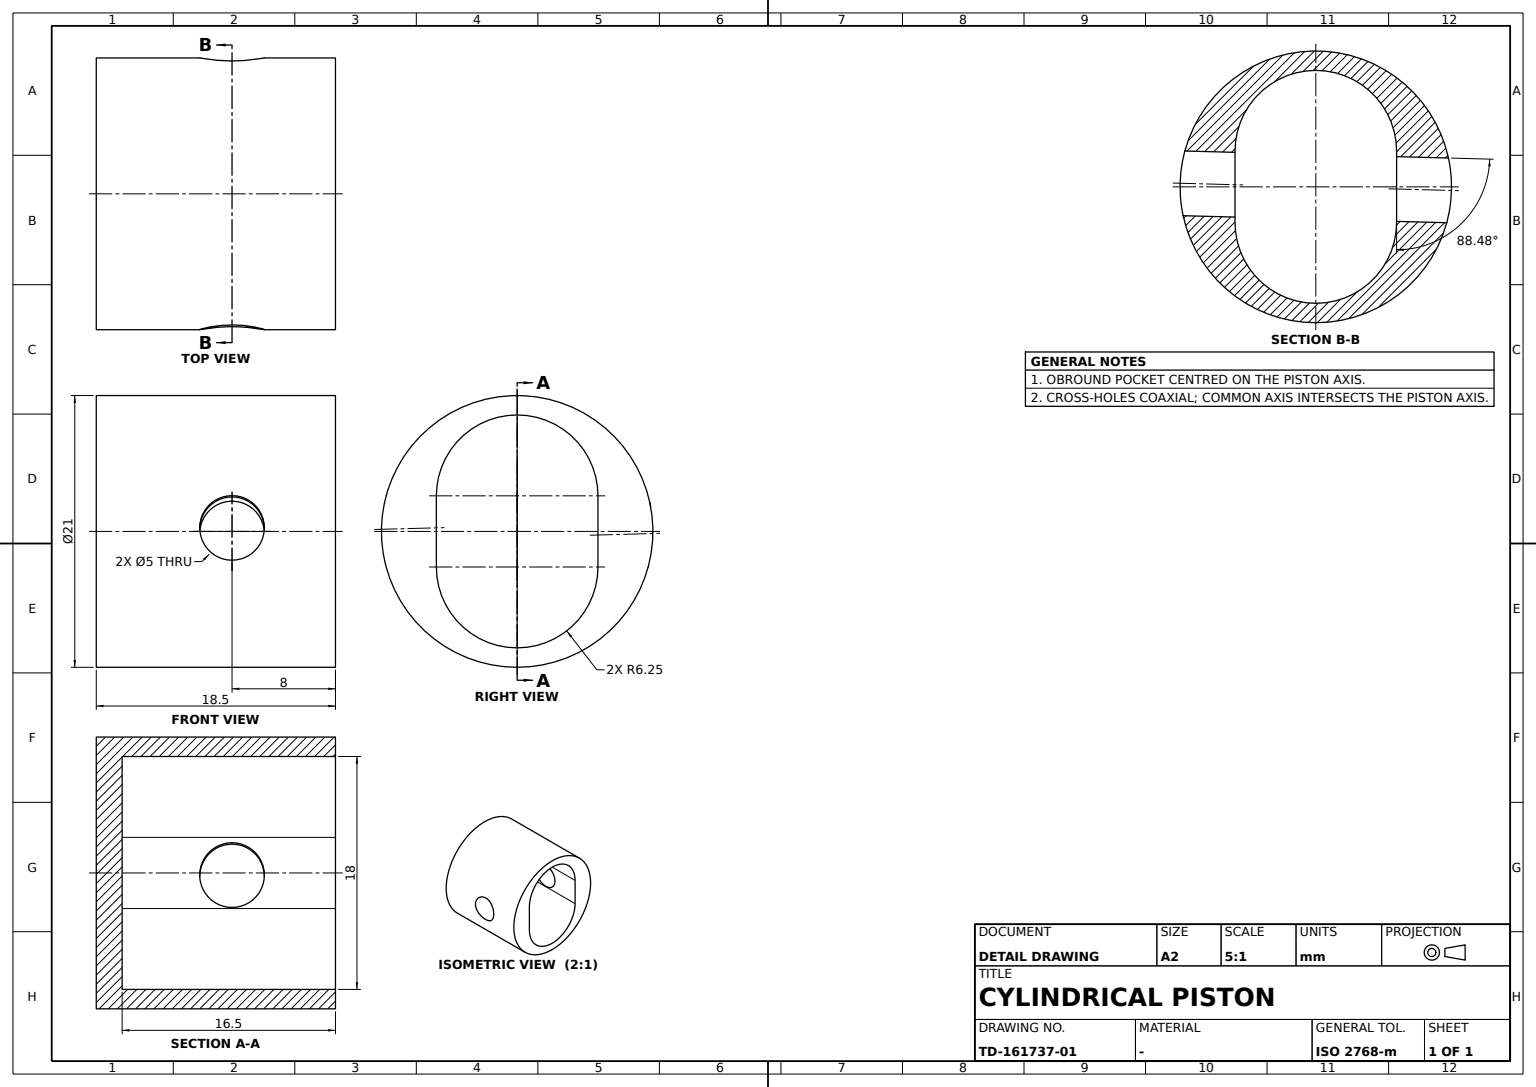
ISO-10303-21;
HEADER;
FILE_DESCRIPTION((''),'2;1');
FILE_NAME('','',(''),(''),'','','');
FILE_SCHEMA(('AUTOMOTIVE_DESIGN'));
ENDSEC;
DATA;
#1=APPLICATION_CONTEXT('');
#2=PRODUCT_CONTEXT('',#1,'mechanical');
#3=PRODUCT('','','',(#2));
#4=PRODUCT_DEFINITION_FORMATION('','',#3);
#5=PRODUCT_DEFINITION_CONTEXT('',#1,'design');
#6=PRODUCT_DEFINITION('','',#4,#5);
#7=PRODUCT_DEFINITION_SHAPE('','',#6);
#8=(LENGTH_UNIT()NAMED_UNIT(*)SI_UNIT(.MILLI.,.METRE.));
#9=(NAMED_UNIT(*)PLANE_ANGLE_UNIT()SI_UNIT($,.RADIAN.));
#10=(NAMED_UNIT(*)SI_UNIT($,.STERADIAN.)SOLID_ANGLE_UNIT());
#11=UNCERTAINTY_MEASURE_WITH_UNIT(LENGTH_MEASURE(0.005),#8,'distance_accuracy_value','');
#12=(GEOMETRIC_REPRESENTATION_CONTEXT(3)GLOBAL_UNCERTAINTY_ASSIGNED_CONTEXT((#11))GLOBAL_UNIT_ASSIGNED_CONTEXT((#8,#9,#10))REPRESENTATION_CONTEXT('',''));
#13=CARTESIAN_POINT('',(-2.75,6.25,-16.5));
#14=VERTEX_POINT('',#13);
#15=CARTESIAN_POINT('',(-2.75,-6.25,-16.5));
#16=VERTEX_POINT('',#15);
#17=CARTESIAN_POINT('',(-2.75,0.,-16.5));
#18=DIRECTION('',(0.,0.,1.));
#19=DIRECTION('',(1.,0.,0.));
#20=AXIS2_PLACEMENT_3D('',#17,#18,#19);
#21=CIRCLE('',#20,6.25);
#22=EDGE_CURVE('',#14,#16,#21,.T.);
#23=ORIENTED_EDGE('',*,*,#22,.F.);
#24=CARTESIAN_POINT('',(-2.75,6.25,0.));
#25=VERTEX_POINT('',#24);
#26=CARTESIAN_POINT('',(-2.75,6.25,-8.25));
#27=VECTOR('',#18,1000.);
#28=LINE('',#26,#27);
#29=EDGE_CURVE('',#25,#14,#28,.F.);
#30=ORIENTED_EDGE('',*,*,#29,.F.);
#31=CARTESIAN_POINT('',(-2.75,-6.25,0.));
#32=VERTEX_POINT('',#31);
#33=CARTESIAN_POINT('',(-2.75,0.,0.));
#34=AXIS2_PLACEMENT_3D('',#33,#18,#19);
#35=CIRCLE('',#34,6.25);
#36=EDGE_CURVE('',#25,#32,#35,.T.);
#37=ORIENTED_EDGE('',*,*,#36,.T.);
#38=CARTESIAN_POINT('',(-2.75,-6.25,-8.25));
#39=LINE('',#38,#27);
#40=EDGE_CURVE('',#32,#16,#39,.F.);
#41=ORIENTED_EDGE('',*,*,#40,.T.);
#42=EDGE_LOOP('',(#23,#30,#37,#41));
#43=FACE_BOUND('',#42,.T.);
#44=CARTESIAN_POINT('',(-2.75,0.,-8.25));
#45=DIRECTION('',(0.,1.,0.));
#46=AXIS2_PLACEMENT_3D('',#44,#18,#45);
#47=CYLINDRICAL_SURFACE('',#46,6.25);
#48=ADVANCED_FACE('',(#43),#47,.F.);
#49=CARTESIAN_POINT('',(1.920707,-10.322833,-6.801436));
#50=VERTEX_POINT('',#49);
#51=CARTESIAN_POINT('',(-2.925057,-10.084733,-7.211843));
#52=CARTESIAN_POINT('',(-2.700374,-10.159778,-9.330518));
#53=CARTESIAN_POINT('',(-1.068055,-10.514373,-10.656274));
#54=CARTESIAN_POINT('',(1.05405,-10.504105,-10.429089));
#55=CARTESIAN_POINT('',(2.385019,-10.225752,-8.788304));
#56=CARTESIAN_POINT('',(2.158084,-10.288764,-6.669213));
#57=CARTESIAN_POINT('',(0.507217,-10.556131,-5.344056));
#58=CARTESIAN_POINT('',(-1.606407,-10.43384,-5.569239));
#59=B_SPLINE_CURVE_WITH_KNOTS('',3,(#51,#52,#53,#54,#55,#56,#57,#58,#51,#52,#53),.UNSPECIFIED.,.T.,.F.,(1,1,1,1,1,1,1,1,1,1,1,1,1,1,1),(-0.005880254,-0.003920244,-0.001960234,-0.000000224,0.001959785,0.003919795,0.005879805,0.007839815,0.009799825,0.011759835,0.013719845,0.015679855,0.017639864,0.019599874,0.021559884),.UNSPECIFIED.);
#60=EDGE_CURVE('',#50,#50,#59,.T.);
#61=ORIENTED_EDGE('',*,*,#60,.T.);
#62=EDGE_LOOP('',(#61));
#63=FACE_BOUND('',#62,.T.);
#64=CARTESIAN_POINT('',(-2.666788,-6.25,-8.));
#65=VERTEX_POINT('',#64);
#66=CARTESIAN_POINT('',(-0.165908,-6.25,-8.));
#67=DIRECTION('',(0.,-1.,0.));
#68=DIRECTION('',(-1.,0.,0.));
#69=AXIS2_PLACEMENT_3D('',#66,#67,#68);
#70=ELLIPSE('',#69,2.500881,2.5);
#71=EDGE_CURVE('',#65,#65,#70,.T.);
#72=ORIENTED_EDGE('',*,*,#71,.F.);
#73=EDGE_LOOP('',(#72));
#74=FACE_BOUND('',#73,.T.);
#75=CARTESIAN_POINT('',(0.275973,10.396338,-8.));
#76=DIRECTION('',(-0.026535879,-0.999647862,0.));
#77=DIRECTION('',(0.999647862,-0.026535879,0.));
#78=AXIS2_PLACEMENT_3D('',#75,#76,#77);
#79=CYLINDRICAL_SURFACE('',#78,2.5);
#80=ADVANCED_FACE('',(#63,#74),#79,.F.);
#81=CARTESIAN_POINT('',(2.75,6.25,-16.5));
#82=VERTEX_POINT('',#81);
#83=VECTOR('',#19,1000.);
#84=LINE('',#13,#83);
#85=EDGE_CURVE('',#14,#82,#84,.T.);
#86=ORIENTED_EDGE('',*,*,#85,.T.);
#87=CARTESIAN_POINT('',(2.75,6.25,0.));
#88=VERTEX_POINT('',#87);
#89=CARTESIAN_POINT('',(2.75,6.25,-8.25));
#90=LINE('',#89,#27);
#91=EDGE_CURVE('',#88,#82,#90,.F.);
#92=ORIENTED_EDGE('',*,*,#91,.F.);
#93=LINE('',#24,#83);
#94=EDGE_CURVE('',#25,#88,#93,.T.);
#95=ORIENTED_EDGE('',*,*,#94,.F.);
#96=ORIENTED_EDGE('',*,*,#29,.T.);
#97=EDGE_LOOP('',(#86,#92,#95,#96));
#98=FACE_BOUND('',#97,.T.);
#99=CARTESIAN_POINT('',(-2.334973,6.25,-8.));
#100=VERTEX_POINT('',#99);
#101=CARTESIAN_POINT('',(0.165908,6.25,-8.));
#102=AXIS2_PLACEMENT_3D('',#101,#45,#68);
#103=ELLIPSE('',#102,2.500881,2.5);
#104=EDGE_CURVE('',#100,#100,#103,.F.);
#105=ORIENTED_EDGE('',*,*,#104,.F.);
#106=EDGE_LOOP('',(#105));
#107=FACE_BOUND('',#106,.T.);
#108=AXIS2_PLACEMENT_3D('',#24,#45,#19);
#109=PLANE('',#108);
#110=ADVANCED_FACE('',(#98,#107),#109,.F.);
#111=CARTESIAN_POINT('',(2.75,-6.25,-16.5));
#112=VERTEX_POINT('',#111);
#113=CARTESIAN_POINT('',(2.75,0.,-16.5));
#114=AXIS2_PLACEMENT_3D('',#113,#18,#19);
#115=CIRCLE('',#114,6.25);
#116=EDGE_CURVE('',#112,#82,#115,.T.);
#117=ORIENTED_EDGE('',*,*,#116,.T.);
#118=ORIENTED_EDGE('',*,*,#85,.F.);
#119=ORIENTED_EDGE('',*,*,#22,.T.);
#120=VECTOR('',#68,1000.);
#121=LINE('',#111,#120);
#122=EDGE_CURVE('',#112,#16,#121,.T.);
#123=ORIENTED_EDGE('',*,*,#122,.F.);
#124=EDGE_LOOP('',(#117,#118,#119,#123));
#125=FACE_BOUND('',#124,.T.);
#126=CARTESIAN_POINT('',(0.,0.,-16.5));
#127=AXIS2_PLACEMENT_3D('',#126,#18,#45);
#128=PLANE('',#127);
#129=ADVANCED_FACE('',(#125),#128,.T.);
#130=CARTESIAN_POINT('',(-1.920707,10.322833,-9.198564));
#131=VERTEX_POINT('',#130);
#132=CARTESIAN_POINT('',(-0.5049,10.556232,-10.656594));
#133=CARTESIAN_POINT('',(-2.158569,10.288769,-9.330532));
#134=CARTESIAN_POINT('',(-2.385067,10.225689,-7.212663));
#135=CARTESIAN_POINT('',(-1.054372,10.504145,-5.570665));
#136=CARTESIAN_POINT('',(1.069219,10.514263,-5.343838));
#137=CARTESIAN_POINT('',(2.700112,10.159792,-6.670487));
#138=CARTESIAN_POINT('',(2.92583,10.084575,-8.78566));
#139=CARTESIAN_POINT('',(1.606161,10.433779,-10.430934));
#140=B_SPLINE_CURVE_WITH_KNOTS('',3,(#132,#133,#134,#135,#136,#137,#138,#139,#132,#133,#134),.UNSPECIFIED.,.T.,.F.,(1,1,1,1,1,1,1,1,1,1,1,1,1,1,1),(-0.005884119,-0.003922746,-0.001961373,0.,0.001961373,0.003922746,0.005884119,0.007845492,0.009806865,0.011768238,0.013729611,0.015690984,0.017652358,0.019613731,0.021575104),.UNSPECIFIED.);
#141=EDGE_CURVE('',#131,#131,#140,.T.);
#142=ORIENTED_EDGE('',*,*,#141,.F.);
#143=EDGE_LOOP('',(#142));
#144=FACE_BOUND('',#143,.T.);
#145=CARTESIAN_POINT('',(10.5,0.,-18.5));
#146=VERTEX_POINT('',#145);
#147=CARTESIAN_POINT('',(0.,0.,-18.5));
#148=AXIS2_PLACEMENT_3D('',#147,#18,#19);
#149=CIRCLE('',#148,10.5);
#150=EDGE_CURVE('',#146,#146,#149,.T.);
#151=ORIENTED_EDGE('',*,*,#150,.T.);
#152=EDGE_LOOP('',(#151));
#153=FACE_BOUND('',#152,.T.);
#154=CARTESIAN_POINT('',(10.5,0.,0.));
#155=VERTEX_POINT('',#154);
#156=CARTESIAN_POINT('',(0.,0.,0.));
#157=AXIS2_PLACEMENT_3D('',#156,#18,#19);
#158=CIRCLE('',#157,10.5);
#159=EDGE_CURVE('',#155,#155,#158,.T.);
#160=ORIENTED_EDGE('',*,*,#159,.F.);
#161=EDGE_LOOP('',(#160));
#162=FACE_BOUND('',#161,.T.);
#163=ORIENTED_EDGE('',*,*,#60,.F.);
#164=EDGE_LOOP('',(#163));
#165=FACE_BOUND('',#164,.T.);
#166=CARTESIAN_POINT('',(0.,0.,-9.25));
#167=AXIS2_PLACEMENT_3D('',#166,#18,#45);
#168=CYLINDRICAL_SURFACE('',#167,10.5);
#169=ADVANCED_FACE('',(#144,#153,#162,#165),#168,.T.);
#170=ORIENTED_EDGE('',*,*,#159,.T.);
#171=EDGE_LOOP('',(#170));
#172=FACE_BOUND('',#171,.T.);
#173=CARTESIAN_POINT('',(2.75,-6.25,0.));
#174=VERTEX_POINT('',#173);
#175=CARTESIAN_POINT('',(2.75,0.,0.));
#176=AXIS2_PLACEMENT_3D('',#175,#18,#19);
#177=CIRCLE('',#176,6.25);
#178=EDGE_CURVE('',#174,#88,#177,.T.);
#179=ORIENTED_EDGE('',*,*,#178,.F.);
#180=LINE('',#173,#120);
#181=EDGE_CURVE('',#174,#32,#180,.T.);
#182=ORIENTED_EDGE('',*,*,#181,.T.);
#183=ORIENTED_EDGE('',*,*,#36,.F.);
#184=ORIENTED_EDGE('',*,*,#94,.T.);
#185=EDGE_LOOP('',(#179,#182,#183,#184));
#186=FACE_BOUND('',#185,.T.);
#187=AXIS2_PLACEMENT_3D('',#156,#18,#45);
#188=PLANE('',#187);
#189=ADVANCED_FACE('',(#172,#186),#188,.T.);
#190=ORIENTED_EDGE('',*,*,#150,.F.);
#191=EDGE_LOOP('',(#190));
#192=FACE_BOUND('',#191,.T.);
#193=AXIS2_PLACEMENT_3D('',#147,#18,#45);
#194=PLANE('',#193);
#195=ADVANCED_FACE('',(#192),#194,.F.);
#196=ORIENTED_EDGE('',*,*,#104,.T.);
#197=EDGE_LOOP('',(#196));
#198=FACE_BOUND('',#197,.T.);
#199=ORIENTED_EDGE('',*,*,#141,.T.);
#200=EDGE_LOOP('',(#199));
#201=FACE_BOUND('',#200,.T.);
#202=ADVANCED_FACE('',(#198,#201),#79,.F.);
#203=CARTESIAN_POINT('',(2.75,-6.25,-8.25));
#204=LINE('',#203,#27);
#205=EDGE_CURVE('',#174,#112,#204,.F.);
#206=ORIENTED_EDGE('',*,*,#205,.F.);
#207=ORIENTED_EDGE('',*,*,#178,.T.);
#208=ORIENTED_EDGE('',*,*,#91,.T.);
#209=ORIENTED_EDGE('',*,*,#116,.F.);
#210=EDGE_LOOP('',(#206,#207,#208,#209));
#211=FACE_BOUND('',#210,.T.);
#212=CARTESIAN_POINT('',(2.75,0.,-8.25));
#213=AXIS2_PLACEMENT_3D('',#212,#18,#45);
#214=CYLINDRICAL_SURFACE('',#213,6.25);
#215=ADVANCED_FACE('',(#211),#214,.F.);
#216=ORIENTED_EDGE('',*,*,#71,.T.);
#217=EDGE_LOOP('',(#216));
#218=FACE_BOUND('',#217,.T.);
#219=ORIENTED_EDGE('',*,*,#205,.T.);
#220=ORIENTED_EDGE('',*,*,#122,.T.);
#221=ORIENTED_EDGE('',*,*,#40,.F.);
#222=ORIENTED_EDGE('',*,*,#181,.F.);
#223=EDGE_LOOP('',(#219,#220,#221,#222));
#224=FACE_BOUND('',#223,.T.);
#225=AXIS2_PLACEMENT_3D('',#173,#67,#68);
#226=PLANE('',#225);
#227=ADVANCED_FACE('',(#218,#224),#226,.F.);
#228=CLOSED_SHELL('',(#48,#80,#110,#129,#169,#189,#195,#202,#215,#227));
#229=MANIFOLD_SOLID_BREP('',#228);
#230=ADVANCED_BREP_SHAPE_REPRESENTATION('',(#229),#12);
#231=SHAPE_DEFINITION_REPRESENTATION(#7,#230);
ENDSEC;
END-ISO-10303-21;
